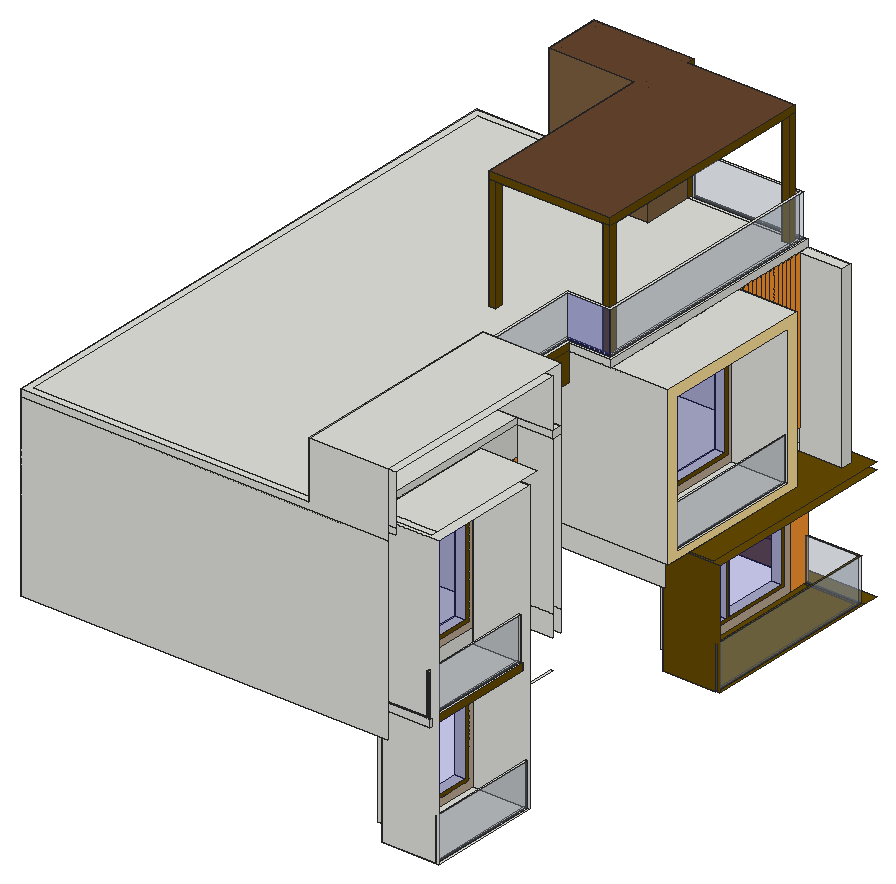
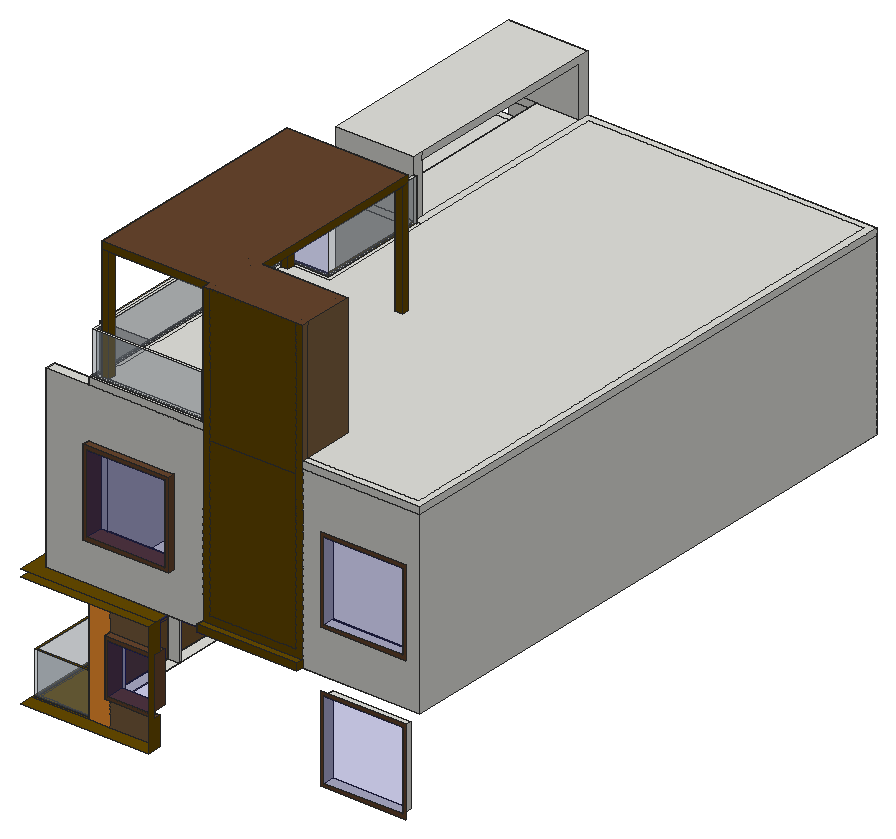
# SketchUp Ruby script. Lengths in inches.
U = 1.inch
M = Sketchup.active_model
def pt(a) = Geom::Point3d.new(a.map { |v| v * U })
def face(e, loops, mat)
  f = e.add_face(loops[0].map { |a| pt(a) })
  loops[1..].each { |l| e.add_face(l.map { |a| pt(a) }).erase! }
  f.material = f.back_material = mat if mat
  f
end
# faces: each face lists its corners as indices into pts; further lists are holes
def faces(e, pts, list, mat = nil) = list.each { |f| face(e, (f[0].is_a?(Array) ? f : [f]).map { |l| l.map { |i| pts[i] } }, mat) }
# xy, xz, yz: faces in a plane at the given z, y or x. An outline is a flat list of corners, or four numbers for a rectangle; further outlines are holes
def ring(l) = l.size == 4 ? [[l[0], l[1]], [l[2], l[1]], [l[2], l[3]], [l[0], l[3]]] : l.each_slice(2).to_a
def flat(e, list, mat, &to3) = list.each { |f| face(e, (f[0].is_a?(Array) ? f : [f]).map { |l| ring(l).map { |u, v| to3.(u, v) } }, mat) }
def xy(e, z, list, mat = nil) = flat(e, list, mat) { |x, y| [x, y, z] }
def xz(e, y, list, mat = nil) = flat(e, list, mat) { |x, z| [x, y, z] }
def yz(e, x, list, mat = nil) = flat(e, list, mat) { |y, z| [x, y, z] }
def lines(e, pts, list) = list.each { |a, b| e.add_line(pt(pts[a]), pt(pts[b])) }
# prism: a flat outline (further loops are holes) pulled along v
def prism(e, loops, v, mat = nil)
  f = face(e, loops, mat); d = Geom::Vector3d.new(v.map { |x| x * U })
  f.pushpull(f.normal.samedirection?(d) ? d.length : -d.length)
end
def box(e, o, s, mat = nil) = prism(e, [[o, [o[0] + s[0], o[1], o[2]], [o[0] + s[0], o[1] + s[1], o[2]], [o[0], o[1] + s[1], o[2]]]], [0, 0, s[2]], mat)
def at(x, y, z, deg = 0) = Geom::Transformation.translation(pt([x, y, z])) * Geom::Transformation.rotation(ORIGIN, Z_AXIS, deg.degrees)
def axes(o, x, y, z) = Geom::Transformation.new([*x, 0, *y, 0, *z, 0, *pt(o).to_a, 1])
def part(name) = M.definitions.add(name)
# library, detail: a bought-in or finely detailed component or shape, given as its bounding box
def library(name, o, s) = part(name).tap { |d| box(d.entities, o, s) }
def detail(e, o, s) = box(e.add_group.entities, o, s)
def put(e, d, t, mat = nil) = e.add_instance(d, t).tap { |i| i.material = mat if mat }
def group(e, t, mat = nil) = e.add_group.tap { |g| g.transformation = t; g.material = mat if mat }.entities
root = M.entities
M.materials.add("C04_Amber_Sunshine").color = [255, 152, 49]
M.materials.add("D02_Buttercup_Glow").color = [255, 229, 155]
M.materials.add("D08_Bronzed_Mustard").color = [102, 74, 0]
M.materials.add("Glass_Basic_01").color = [161, 173, 186]
M.materials["Glass_Basic_01"].alpha = 0.25
M.materials.add("Glass_Sky Reflection_1").color = [0, 2, 183]
M.materials["Glass_Sky Reflection_1"].alpha = 0.25
M.materials.add("Plywood_01_1K").color = [125, 96, 64]
M.materials.add("ThomThom - Complexion1").color = [190, 169, 148]
M.materials.add("Wood_Veneer_15_1K").color = [103, 69, 45]
xy(root,570,[[279,43.85,322.5,139.15],[322.5,43.85,324,139.15],[325.5,43.85,327,139.15]])
xy(root,570,[[279,339,322.5,339,322.5,343.5,283.5,343.5,283.5,487.5,279,487.5],[322.5,339,324,339,324,489,279,489,279,487.5,322.5,487.5],[325.5,339,327,339,327,492,279,492,279,490.5,325.5,490.5],[283.5,343.5,322.5,487.5],[219,492,327,504]],"D08_Bronzed_Mustard")
xy(root,576,[[228,195,229.5,285]])
xy(root,579,[[270,51,279,89.5],[270,91.5,279,132],[270,348,279,406.5],[270,408.5,279,465]])
xy(root,591,[[15,483,81,492]])
xy(root,594,[[219,492,261,498]],"Wood_Veneer_15_1K")
xy(root,597,[[222,483,258,498]],"Wood_Veneer_15_1K")
xy(root,606,[[324,43.85,325.5,139.15]])
xy(root,606,[[324,339,325.5,339,325.5,490.5,279,490.5,279,489,324,489]],"D08_Bronzed_Mustard")
xy(root,633,[[192,240,201,270]])
xy(root,639,[[222,483,258,498]],"Wood_Veneer_15_1K")
xy(root,642,[[219,492,261,498]],"Wood_Veneer_15_1K")
xy(root,645,[[270,51,279,89.5],[270,91.5,279,132]])
xy(root,657,[[270,348,279,406.5],[270,408.5,279,465],[15,483,81,492]])
xy(root,666,[[279,339,279,492,219,492,219,504,327,504,327,339]],"D08_Bronzed_Mustard")
xy(root,672,[[0,12,9,492],[9,21,9,483,192,483,192,186,270,186,270,21],[279,42,321,43.85],[279,139.15,321,141],[201,195,201,285,234,285,234,281.5,237,281.5,237,278,234,278,234,274.5,237,274.5,237,271,234,271,234,267.5,237,267.5,237,264,234,264,234,260.5,237,260.5,237,257,234,257,234,253.5,237,253.5,237,250,234,250,234,246.5,237,246.5,237,195],
  [192,294,270,483],[9,483,192,492],[192,483,279,492]])
xy(root,672,[[279,43.85,321,139.15],[279,333,327,333,327,504,213,504,213,492,315,492,315,483,279,483],[99,492,183,498]],"D08_Bronzed_Mustard")
xy(root,678,[[9,21,270,21,270,186,192,186,192,294,270,294,270,483,9,483],[279,42,316.5,43.85],[316.5,42,318,43.85],[319.5,42,321,43.85],[279,43.85,316.5,139.15],
  [316.5,43.85,318,139.15],[319.5,43.85,321,139.15],[279,139.15,316.5,141],[316.5,139.15,318,141],[319.5,139.15,321,141],
  [201,195,226.5,285]])
xy(root,678,[[99,492,183,498]],"D08_Bronzed_Mustard")
xy(root,681,[[192,240,201,270]])
xy(root,690,[[226.5,195,228,285],[229.5,195,237,195,237,198.5,234,198.5,234,237,237,237,237,285,229.5,285],[234,202,237,205.5],[234,209,237,212.5],[234,216,237,219.5],
  [234,223,237,226.5],[234,230,237,233.5],[324,285,327,291],[279,291,327,420]])
xy(root,696,[[279,294,322.5,411],[322.5,294,324,411],[325.5,294,327,411]])
xy(root,699,[[270,51,279,89.5],[270,91.5,279,132]])
xy(root,702,[[228,195,229.5,285]])
xy(root,705,[[270,300,279,352.5],[270,354.5,279,405]])
xy(root,708,[[207,492,279,498]],"Wood_Veneer_15_1K")
xy(root,711,[[15,483,81,492]])
xy(root,711,[[210,483,276,498]],"Wood_Veneer_15_1K")
xy(root,714,[[318,42,319.5,43.85],[318,43.85,319.5,139.15],[318,139.15,319.5,141]])
xy(root,732,[[324,294,325.5,411]])
xy(root,759,[[192,240,201,270]])
xy(root,777,[[15,483,81,492]])
xy(root,777,[[210,483,276,498]],"Wood_Veneer_15_1K")
xy(root,780,[[207,492,279,498]],"Wood_Veneer_15_1K")
xy(root,789,[[270,51,279,89.5],[270,91.5,279,132]])
xy(root,798,[[[201,195,243,285],[234,198.5,237,202],[234,205.5,237,209],[234,212.5,237,216],[234,219.5,237,223],[234,226.5,237,230],[234,233.5,237,237]]])
xy(root,807,[[270,300,279,352.5],[270,354.5,279,405]])
xy(root,813,[[279,294,327,411]])
xy(root,814.15,[[279,43.85,327,139.15]])
xy(root,822,[[0,12,270,21],[0,21,9,492],[9,21,9,483,192,483,192,186,270,186,270,21],[279,36,327,42],[279,42,327,147],
  [192,186,192,294,279,294,279,285,243,285,243,195,270,195,270,186],[279,285,327,420],[192,294,270,483],[270,294,279,483],[192,483,279,492],
  [279,483,315,492]])
xy(root,828,[[0,12,243,12,243,195,237,195,237,18,6,18,6,486,99,486,99,492,0,492],[6,18,237,18,237,291,267,291,267,297,273,297,273,480,267,480,267,486,183,486,183,444,99,444,99,486,6,486],[243,21,279,186],[243,186,309,195],[[237,195,243,195,243,285,279,285,279,492,183,492,183,486,273,486,273,291,237,291],[239,197,239,289,275,289,275,488,185,488,185,490,277,490,277,287,241,287,241,197]],
  [105,450,177,486]])
xy(root,864,[[239,197,241,197,241,287,277,287,277,490,185,490,185,488,275,488,275,289,239,289]])
xy(root,870,[[243,21,309,186]])
xy(root,876,[[243,12,309,195]])
xy(root,924,[[171,291,177,297],[267,291,273,297],[267,480,273,486]])
xy(root,924,[[177,291,177,297,171,297,171,444,183,444,183,486,267,486,267,480,273,480,273,297,267,297,267,291]],"D08_Bronzed_Mustard")
xy(root,930,[[171,291,273,291,273,486,183,486,183,492,99,492,99,444,171,444]],"Wood_Veneer_15_1K")
xz(root,12,[[0,672,309,822],[0,822,309,822,309,876,243,876,243,828,0,828]])
xz(root,21,[[9,678,270,822],[279,822,309,828],[243,828,309,870]])
xz(root,42,[[279,672,279,678,318,678,318,714,319.5,714,319.5,678,321,678,321,672]])
xz(root,43.85,[[279,570,279,672,321,672,321,678,319.5,678,319.5,714,318,714,318,678,279,678,279,814.15,327,814.15,327,570,325.5,570,325.5,606,324,606,324,570]])
xz(root,51,[[270,579,279,645],[270,699,279,789]])
xz(root,89.5,[[270,579,279,645],[270,699,279,789]])
xz(root,91.5,[[270,579,279,645],[270,699,279,789]])
xz(root,132,[[270,579,279,645],[270,699,279,789]])
xz(root,139.15,[[279,570,324,570,324,606,325.5,606,325.5,570,327,570,327,814.15,279,814.15,279,678,318,678,318,714,319.5,714,319.5,678,321,678,321,672,279,672]])
xz(root,141,[[279,672,321,672,321,678,319.5,678,319.5,714,318,714,318,678,279,678]])
xz(root,186,[[279,672,309,690],[192,678,270,822],[279,690,309,822],[279,822,309,828],[243,828,309,870]])
xz(root,195,[[237,672,309,690],[201,678,226.5,690],[201,690,201,798,243,798,243,822,309,822,309,690,229.5,690,229.5,702,228,702,228,690],[243,822,309,828],[243,828,309,876]])
xz(root,197,[[239,828,241,864]])
xz(root,198.5,[[234,690,237,798]])
xz(root,202,[[234,690,237,798]])
xz(root,205.5,[[234,690,237,798]])
xz(root,209,[[234,690,237,798]])
xz(root,212.5,[[234,690,237,798]])
xz(root,216,[[234,690,237,798]])
xz(root,219.5,[[234,690,237,798]])
xz(root,223,[[234,690,237,798]])
xz(root,226.5,[[234,690,237,798]])
xz(root,230,[[234,690,237,798]])
xz(root,233.5,[[234,690,237,798]])
xz(root,237,[[234,690,237,798]])
xz(root,240,[[192,681,201,759]])
xz(root,270,[[192,681,201,759]])
xz(root,285,[[237,672,324,690],[201,678,226.5,690],[201,690,228,690,228,702,229.5,702,229.5,690,327,690,327,822,243,822,243,798,201,798],[243,822,279,828]])
xz(root,287,[[241,828,277,864]],"Glass_Sky Reflection_1")
xz(root,289,[[239,828,275,864]],"Glass_Basic_01")
xz(root,291,[[171,828,177,924],[267,828,273,924],[171,924,273,930]],"D08_Bronzed_Mustard")
xz(root,294,[[192,678,270,822],[279,696,279,813,327,813,327,696,325.5,696,325.5,732,324,732,324,696]])
xz(root,297,[[171,828,177,924],[267,828,273,924]],"D08_Bronzed_Mustard")
xz(root,300,[[270,705,279,807]])
xz(root,339,[[279,570,279,666,327,666,327,570,325.5,570,325.5,606,324,606,324,570]],"D08_Bronzed_Mustard")
xz(root,348,[[270,579,279,657]])
xz(root,352.5,[[270,705,279,807]])
xz(root,354.5,[[270,705,279,807]])
xz(root,405,[[270,705,279,807]])
xz(root,406.5,[[270,579,279,657]])
xz(root,408.5,[[270,579,279,657]])
xz(root,411,[[279,696,324,696,324,732,325.5,732,325.5,696,327,696,327,813,279,813]])
xz(root,420,[[279,690,327,822]])
xz(root,444,[[99,828,183,828,183,924,171,924,171,930,99,930]],"Plywood_01_1K")
xz(root,465,[[270,579,279,657]])
xz(root,480,[[267,828,273,924]],"D08_Bronzed_Mustard")
xz(root,483,[[279,672,315,822],[[9,678,270,678,270,711,210,711,210,777,270,777,270,822,9,822],[15,711,81,777]],[270,711,276,777]])
xz(root,486,[[99,828,105,924]])
xz(root,486,[[267,828,273,924],[183,924,273,930]],"D08_Bronzed_Mustard")
xz(root,488,[[185,828,275,864]],"Glass_Basic_01")
xz(root,489,[[279,570,324,606]],"Glass_Basic_01")
xz(root,490,[[185,828,277,864]],"Glass_Basic_01")
xz(root,490.5,[[279,570,325.5,606]],"Glass_Basic_01")
xz(root,492,[[[0,672,99,822],[12,708,84,780]],[[183,672,315,822],[207,708,279,780]],[0,822,99,828],[183,822,279,828]])
xz(root,492,[[261,570,279,666]],"C04_Amber_Sunshine")
xz(root,492,[[99,678,99,930,105,930,105,684,177,684,177,930,183,930,183,678],[105,684,177,816],[105,816,177,930]],"D08_Bronzed_Mustard")
xz(root,492,[[15,591,81,657],[15,711,81,777]],"Glass_Sky Reflection_1")
xz(root,492,[[219,570,261,594],[219,642,261,666]],"Plywood_01_1K")
xz(root,492,[[[12,588,84,660],[15,591,81,657]],[[12,708,84,780],[15,711,81,777]]],"Wood_Veneer_15_1K")
xz(root,498,[[99,672,183,678]],"D08_Bronzed_Mustard")
xz(root,498,[[222,597,258,639],[210,711,276,777]],"Glass_Sky Reflection_1")
xz(root,498,[[[219,594,261,642],[222,597,258,639]],[[207,708,279,780],[210,711,276,777]]],"Wood_Veneer_15_1K")
yz(root,0,[[12,672,492,822],[12,822,492,828]])
yz(root,9,[[21,678,483,822]])
yz(root,15,[[483,591,492,657],[483,711,492,777]])
yz(root,81,[[483,591,492,657],[483,711,492,777]])
yz(root,99,[[492,672,498,678]],"D08_Bronzed_Mustard")
yz(root,99,[[444,828,486,930],[486,828,492,930]],"Plywood_01_1K")
yz(root,171,[[291,828,297,924],[291,924,444,930]],"D08_Bronzed_Mustard")
yz(root,177,[[291,828,297,924]],"D08_Bronzed_Mustard")
yz(root,183,[[492,672,498,678],[486,828,492,930]],"D08_Bronzed_Mustard")
yz(root,183,[[444,828,486,924]],"Plywood_01_1K")
yz(root,185,[[488,828,490,864]])
yz(root,192,[[[186,678,294,822],[240,681,270,759]]])
yz(root,201,[[195,678,237,678,237,762,273,762,273,678,285,678,285,798,195,798]])
yz(root,201,[[[237,678,273,762],[240,681,270,759]]],"D08_Bronzed_Mustard")
yz(root,207,[[492,708,498,780]],"Wood_Veneer_15_1K")
yz(root,210,[[483,711,498,777]],"Wood_Veneer_15_1K")
yz(root,219,[[492,570,504,570,504,666,492,666,492,642,498,642,498,594,492,594]],"D08_Bronzed_Mustard")
yz(root,222,[[483,597,498,639]],"Wood_Veneer_15_1K")
yz(root,226.5,[[195,678,285,690]])
yz(root,228,[[195,690,285,702]],"Glass_Basic_01")
yz(root,229.5,[[195,690,285,702]],"Glass_Basic_01")
yz(root,234,[[198.5,690,202,798],[205.5,690,209,798],[212.5,690,216,798],[219.5,690,223,798],[226.5,690,230,798],
  [233.5,690,237,798]])
yz(root,237,[[195,672,198.5,690],[198.5,672,202,798],[202,672,205.5,690],[205.5,672,209,798],[209,672,212.5,690],
  [212.5,672,216,798],[216,672,219.5,690],[219.5,672,223,798],[223,672,226.5,690],[226.5,672,230,798],
  [230,672,233.5,690],[233.5,672,237,798],[237,672,285,690]],"D08_Bronzed_Mustard")
yz(root,239,[[197,828,289,864]],"Glass_Basic_01")
yz(root,241,[[197,828,287,864]],"Glass_Basic_01")
yz(root,243,[[12,828,12,876,186,876,186,870,21,870,21,828],[186,828,195,876]])
yz(root,243,[[195,798,285,822],[195,822,285,828]],"D08_Bronzed_Mustard")
yz(root,258,[[483,597,498,639]],"Wood_Veneer_15_1K")
yz(root,261,[[492,594,498,642]],"Wood_Veneer_15_1K")
yz(root,267,[[291,828,297,924],[480,828,486,924]],"D08_Bronzed_Mustard")
yz(root,270,[[[21,678,186,822],[91.5,699,132,789],[51,699,89.5,789]],[[294,678,483,822],[300,705,352.5,807],[354.5,705,405,807]]])
yz(root,273,[[291,828,297,924],[480,828,486,924],[291,924,486,930]],"D08_Bronzed_Mustard")
yz(root,275,[[289,828,488,864]],"Glass_Basic_01")
yz(root,276,[[483,711,498,777]],"Wood_Veneer_15_1K")
yz(root,277,[[287,828,490,864]],"Glass_Basic_01")
yz(root,279,[[36,672,42,672,42,678,43.85,678,43.85,816,42,816,42,822,36,822],[141,672,147,672,147,822,141,822,141,816,139.15,816,139.15,678,141,678],[147,672,186,690],[43.85,678,139.15,690],[147,798,186,822],
  [43.85,814.15,139.15,814.15,139.15,816,141,816,141,822,42,822,42,816,43.85,816],[21,822,186,828],[285,822,492,828]])
yz(root,279,[[474,570,489,570,489,606,490.5,606,490.5,570,492,570,492,666,474,666],[147,690,150.9,798],[150.9,690,154.8,798],[154.8,690,158.7,798],[158.7,690,162.6,798],
  [162.6,690,166.5,798],[166.5,690,170.4,798],[170.4,690,174.3,798],[174.3,690,178.2,798],[178.2,690,182.1,798],
  [182.1,690,186,798],[420,690,424.5,822],[424.5,690,429,822],[429,690,433.5,822],[433.5,690,438,822],
  [438,690,442.5,822],[442.5,690,447,822],[447,690,451.5,822],[451.5,690,456,822],[456,690,460.5,822],
  [460.5,690,465,822],[465,690,469.5,822],[469.5,690,474,822],[474,690,478.5,822],[478.5,690,483,822]],"C04_Amber_Sunshine")
yz(root,279,[[[48,576,135,648],[51,579,51,645,89.5,645,89.5,579,91.5,579,91.5,645,132,645,132,579]],[[345,576,468,660],[348,579,348,657,406.5,657,406.5,579,408.5,579,408.5,657,465,657,465,579]],[[48,696,135,792],[51,699,51,789,132,789,132,699,91.5,699,91.5,789,89.5,789,89.5,699]],[[297,702,408,810],[300,705,300,807,352.5,807,352.5,705,354.5,705,354.5,807,405,807,405,705]]],"D08_Bronzed_Mustard")
yz(root,279,[[51,579,89.5,645],[91.5,579,132,645],[348,579,406.5,657],[408.5,579,465,657],[51,699,89.5,789],
  [91.5,699,132,789],[300,705,352.5,807],[354.5,705,405,807]],"Glass_Sky Reflection_1")
yz(root,279,[[[43.85,570,139.15,654],[48,576,135,648]],[[339,570,474,666],[345,576,468,660]],[43.85,654,139.15,672],[[43.85,690,139.15,798],[48,696,135,792]],[[294,696,411,813],[297,702,408,810]],
  [43.85,798,139.15,814.15]],"ThomThom - Complexion1")
yz(root,279,[[492,708,498,780]],"Wood_Veneer_15_1K")
yz(root,309,[[186,822,195,828]])
yz(root,315,[[483,672,492,822]])
yz(root,318,[[42,678,43.85,714],[139.15,678,141,714]])
yz(root,318,[[43.85,678,139.15,714]],"Glass_Basic_01")
yz(root,319.5,[[42,678,43.85,714],[139.15,678,141,714]])
yz(root,319.5,[[43.85,678,139.15,714]],"Glass_Basic_01")
yz(root,321,[[42,672,43.85,678],[139.15,672,141,678]])
yz(root,321,[[43.85,672,139.15,678]],"D08_Bronzed_Mustard")
yz(root,324,[[43.85,570,139.15,606],[339,570,489,606],[294,696,411,732]],"Glass_Basic_01")
yz(root,325.5,[[43.85,570,139.15,606],[339,570,490.5,606],[294,696,411,732]],"Glass_Basic_01")
yz(root,327,[[[285,690,420,822],[294,696,411,813]]],"D02_Buttercup_Glow")
p = [[279,165,666],[270.1,165,666],[270,21,672],[279,21,672],[270,186,672],[270,195,672],
  [279,294,672],[270,294,672],[234,285,672],[237,285,672],[279,291,696],[279,291,690],
  [177,486,828],[177,486,930],[177,450,828],[177,450,930],[105,450,828],[105,450,930],
  [183,444,924],[183,444,930],[105,486,924],[105,486,930]]
lines(root,p,[[0,1],[2,3],[4,5],[6,7],[8,9],[10,11],[12,13],[14,15],[16,17],[18,19],[20,21]])
